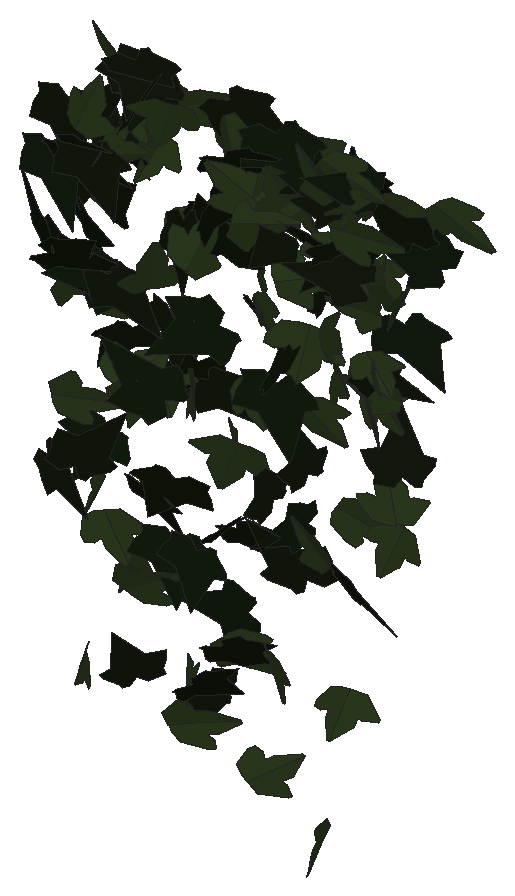
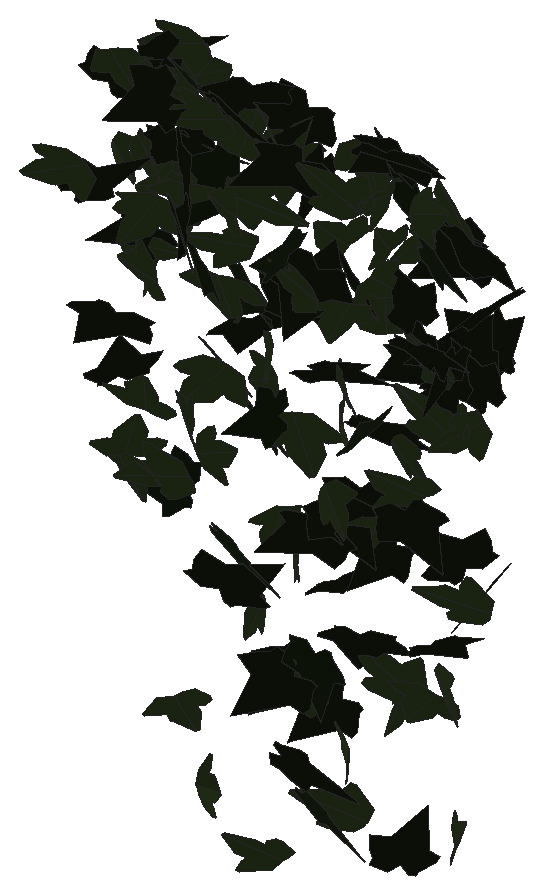
# SketchUp Ruby script. Lengths in inches.
U = 1.inch
M = Sketchup.active_model
def pt(a) = Geom::Point3d.new(a.map { |v| v * U })
def face(e, loops, mat)
  f = e.add_face(loops[0].map { |a| pt(a) })
  loops[1..].each { |l| e.add_face(l.map { |a| pt(a) }).erase! }
  f.material = f.back_material = mat if mat
  f
end
# faces: each face lists its corners as indices into pts; further lists are holes
def faces(e, pts, list, mat = nil) = list.each { |f| face(e, (f[0].is_a?(Array) ? f : [f]).map { |l| l.map { |i| pts[i] } }, mat) }
# xy, xz, yz: faces in a plane at the given z, y or x. An outline is a flat list of corners, or four numbers for a rectangle; further outlines are holes
def ring(l) = l.size == 4 ? [[l[0], l[1]], [l[2], l[1]], [l[2], l[3]], [l[0], l[3]]] : l.each_slice(2).to_a
def flat(e, list, mat, &to3) = list.each { |f| face(e, (f[0].is_a?(Array) ? f : [f]).map { |l| ring(l).map { |u, v| to3.(u, v) } }, mat) }
def xy(e, z, list, mat = nil) = flat(e, list, mat) { |x, y| [x, y, z] }
def xz(e, y, list, mat = nil) = flat(e, list, mat) { |x, z| [x, y, z] }
def yz(e, x, list, mat = nil) = flat(e, list, mat) { |y, z| [x, y, z] }
def lines(e, pts, list) = list.each { |a, b| e.add_line(pt(pts[a]), pt(pts[b])) }
# prism: a flat outline (further loops are holes) pulled along v
def prism(e, loops, v, mat = nil)
  f = face(e, loops, mat); d = Geom::Vector3d.new(v.map { |x| x * U })
  f.pushpull(f.normal.samedirection?(d) ? d.length : -d.length)
end
def box(e, o, s, mat = nil) = prism(e, [[o, [o[0] + s[0], o[1], o[2]], [o[0] + s[0], o[1] + s[1], o[2]], [o[0], o[1] + s[1], o[2]]]], [0, 0, s[2]], mat)
def at(x, y, z, deg = 0) = Geom::Transformation.translation(pt([x, y, z])) * Geom::Transformation.rotation(ORIGIN, Z_AXIS, deg.degrees)
def axes(o, x, y, z) = Geom::Transformation.new([*x, 0, *y, 0, *z, 0, *pt(o).to_a, 1])
def part(name) = M.definitions.add(name)
# library, detail: a bought-in or finely detailed component or shape, given as its bounding box
def library(name, o, s) = part(name).tap { |d| box(d.entities, o, s) }
def detail(e, o, s) = box(e.add_group.entities, o, s)
def put(e, d, t, mat = nil) = e.add_instance(d, t).tap { |i| i.material = mat if mat }
def group(e, t, mat = nil) = e.add_group.tap { |g| g.transformation = t; g.material = mat if mat }.entities
root = M.entities
M.materials.add("1026 AP 7946 SUNNY SIDE UP").color = [254, 231, 186]
M.materials.add("efeu1").color = [18, 25, 13]
M.materials.add("efeu2").color = [43, 57, 29]
c1 = part("ivyleaf_9")
p = [[1.54,2.16,1.25],[1.36,2.04,1.19],[-0.21,0.99,0.68],[-0.71,1.11,0.82],[-0.85,0.86,0.67],[-0.8,0.17,0.21],
  [-0.9,-0.01,0.1],[-0.67,-0.16,-0.02],[-0.08,-0.08,-0.05],[-0.03,-0.6,-0.4],[0.65,-0.88,-0.66],[0.83,-0.6,-0.49],
  [1.29,-0.42,-0.43],[1.8125,-0.07,-0.26],[1.21,0.44,0.15]]
faces(c1.entities,p,[[0,1,2,3,4,5,6,7,8,9,10,11,12,13,14]],"efeu1")
c2 = part("ivyleaf_10")
p = [[0,0.5,-0.03],[-0.0625,2.02,-0.43],[-0.19,2.01,-0.46],[-0.54,1.05,-0.29],[-0.52,0.625,-0.18],[-0.83,0.76,-0.28],
  [-1.16,0.64,-0.33],[-1.15,0.33,-0.24],[-0.77,-0.39,0.02],[-0.3,-0.51,0.16],[0.04,-0.48,0.23],[-0.02,2.01,-0.4375],
  [-0.06,2.01,-0.43],[0.04,-0.49,0.23],[0.67,-0.49,0.14],[1.38,0.36,-0.2],[1.375,0.51,-0.24],[0.81,0.65,-0.19],
  [0.62,0.59,-0.15],[0.6,1.09,-0.28],[0.5,1.23,-0.31]]
faces(c2.entities,p,[[0,1,2,3,4,5,6,7,8,9,10],[11,12,0,13,14,15,16,17,18,19,20]],"efeu2")
put(root,c1,axes([130.41,212.4,265.85],[-0.4161,-0.11399,-0.10586],[0.16625,0.01128,-0.29519],[0.17397,-0.28342,0.0289]),"1026 AP 7946 SUNNY SIDE UP")
put(root,c2,axes([130.06,211.54,261.31],[-0.09725,0.00024,0.32369],[0.41165,0.17712,0.05398],[-0.27319,0.26679,-0.03389]),"1026 AP 7946 SUNNY SIDE UP")
put(root,c1,axes([130.375,211.64,265.35],[0.10675,-0.1348,-0.29209],[-0.24694,0.23569,-0.15322],[0.42618,0.17033,-0.01562]),"1026 AP 7946 SUNNY SIDE UP")
put(root,c1,axes([130.58,210.33,264.84],[0.08748,-0.17485,0.29547],[-0.06631,0.28579,0.18894],[-0.52534,-0.06519,0.02535]),"1026 AP 7946 SUNNY SIDE UP")
put(root,c1,axes([130.27,210.95,265.93],[0.03924,-0.37961,-0.02403],[-0.00771,0.02089,-0.39177],[0.59777,0.02519,-0.00348]),"1026 AP 7946 SUNNY SIDE UP")
put(root,c1,axes([130.53,211.9,260.69],[-0.27687,-0.23897,0.07479],[-0.04522,-0.0705,-0.30564],[0.39072,-0.17749,0.01762]),"1026 AP 7946 SUNNY SIDE UP")
put(root,c2,axes([130.61,211.62,259.94],[0.18156,-0.29153,-0.01318],[-0.02473,0.00574,-0.32274],[0.45807,0.11586,-0.0122]),"1026 AP 7946 SUNNY SIDE UP")
put(root,c1,axes([130.5,211.02,266.875],[-0.3624,-0.07053,-0.28017],[0.42422,0.04074,-0.24655],[0.12108,-0.35384,0.02528]),"1026 AP 7946 SUNNY SIDE UP")
put(root,c2,axes([130.57,210.92,263.8125],[-0.10801,-0.11461,-0.30654],[0.27721,0.23918,-0.13574],[0.41664,-0.18885,0.01084]),"1026 AP 7946 SUNNY SIDE UP")
put(root,c1,axes([130.45,210.83,264.34],[-0.00135,-0.02148,0.32525],[0.23378,-0.27887,-0.02076],[0.43946,0.14828,0.01204]),"1026 AP 7946 SUNNY SIDE UP")
put(root,c2,axes([130.7,211.22,257.11],[-0.00482,0.04885,-0.30958],[0.02814,-0.30025,-0.05218],[-0.47832,-0.01815,0.00005]),"1026 AP 7946 SUNNY SIDE UP")
put(root,c2,axes([131.05,211.57,267.45],[-0.1691,0.14723,-0.26811],[-0.28544,0.18873,0.18778],[0.37504,0.21003,0.02203]),"1026 AP 7946 SUNNY SIDE UP")
put(root,c1,axes([130.53,211.39,264.57],[0.0731,-0.0828,0.29971],[0.1641,-0.27239,-0.09848],[0.44718,0.11349,-0.01286]),"1026 AP 7946 SUNNY SIDE UP")
put(root,c1,axes([130.66,210.38,260.98],[0.26146,-0.24764,-0.17909],[-0.15805,0.14018,-0.30643],[0.44739,0.19425,-0.00359]),"1026 AP 7946 SUNNY SIDE UP")
put(root,c1,axes([130.95,211.57,266.88],[-0.34929,0.13944,-0.16772],[0.18724,-0.11603,-0.26914],[-0.2814,-0.25029,0.02909]),"1026 AP 7946 SUNNY SIDE UP")
put(root,c2,axes([130.54,211.73,265.12],[0.15804,-0.09938,-0.30184],[0.37693,-0.16881,0.14299],[-0.30622,-0.25908,0.02023]),"1026 AP 7946 SUNNY SIDE UP")
put(root,c1,axes([131.03,211.89,262.68],[0.05808,0.21636,-0.21679],[-0.04333,-0.20995,-0.22726],[-0.47395,0.04571,-0.00579]),"1026 AP 7946 SUNNY SIDE UP")
put(root,c1,axes([130.96,211.5,265.05],[-0.0691,0.09761,0.31381],[0.12997,-0.29299,0.10749],[0.48503,0.09241,0.0159]),"1026 AP 7946 SUNNY SIDE UP")
put(root,c1,axes([130.88,210.49,266.46],[0.49526,0.04975,0.08038],[0.12809,-0.01989,-0.32702],[-0.06823,0.32381,-0.03049]),"1026 AP 7946 SUNNY SIDE UP")
put(root,c2,axes([130.93,211.46,259.47],[0.41877,0.11041,0.15008],[0.22928,0.02509,-0.29534],[-0.17203,0.30223,-0.02829]),"1026 AP 7946 SUNNY SIDE UP")
put(root,c1,axes([131.26,211.74,256.79],[0.21556,0.113,0.25928],[-0.36903,-0.09862,0.17719],[0.22627,-0.26849,0.04198]),"1026 AP 7946 SUNNY SIDE UP")
put(root,c2,axes([131.0625,210.69,266.91],[0.48737,-0.17816,-0.02697],[0.06055,0.01671,0.36677],[-0.27636,-0.31052,0.03279]),"1026 AP 7946 SUNNY SIDE UP")
put(root,c1,axes([130.88,210.16,264.72],[0.38747,0.12743,0.2176],[0.31784,0.06505,-0.28396],[-0.22064,0.31749,-0.02692]),"1026 AP 7946 SUNNY SIDE UP")
put(root,c1,axes([130.98,211.77,265.875],[-0.02801,-0.107,0.30558],[0.21146,-0.27195,-0.09414],[0.44947,0.12128,0.06333]),"1026 AP 7946 SUNNY SIDE UP")
put(root,c1,axes([131.41,210.9,264.16],[-0.01935,-0.24901,-0.22279],[0.01795,-0.21519,0.25501],[-0.51683,0.00185,0.0172]),"1026 AP 7946 SUNNY SIDE UP")
put(root,c2,axes([131.03,211.05,263.67],[-0.35983,-0.03803,0.26783],[0.39011,0.08311,0.23778],[-0.13705,0.3364,-0.02636]),"1026 AP 7946 SUNNY SIDE UP")
put(root,c1,axes([131.21,210.36,261.08],[-0.14586,-0.052,0.33939],[0.46342,0.14793,0.11032],[-0.24646,0.30894,0.00657]),"1026 AP 7946 SUNNY SIDE UP")
put(root,c1,axes([131.38,210.45,266.53],[-0.25841,-0.13518,-0.25909],[0.34512,0.1244,-0.21658],[0.28547,-0.27276,0.02731]),"1026 AP 7946 SUNNY SIDE UP")
put(root,c2,axes([131.66,211.14,259.14],[-0.0176,-0.21279,-0.25113],[0.08895,0.23765,-0.21607],[0.4995,-0.04982,0.02963]),"1026 AP 7946 SUNNY SIDE UP")
put(root,c2,axes([131.58,210.65,266.53],[-0.0774,-0.12712,-0.33864],[0.22425,0.29554,-0.13832],[0.50562,-0.15054,0.00951]),"1026 AP 7946 SUNNY SIDE UP")
put(root,c2,axes([131.75,211.73,266.22],[0.14936,0.20643,-0.24394],[-0.14698,-0.21889,-0.23533],[-0.47304,0.13319,-0.0039]),"1026 AP 7946 SUNNY SIDE UP")
put(root,c2,axes([131.74,211.4,266.59],[0.08454,0.22627,-0.21222],[0.07568,0.20162,0.24077],[0.47653,-0.07216,-0.00059]),"1026 AP 7946 SUNNY SIDE UP")
put(root,c2,axes([131.72,211.75,262.2],[0.25185,0.2614,0.02942],[0.04334,0.01482,-0.31532],[-0.41094,0.16176,-0.01523]),"1026 AP 7946 SUNNY SIDE UP")
put(root,c2,axes([131.58,211.03,262.4375],[0.33233,0.0674,-0.27773],[0.32476,0.18919,0.21633],[0.29321,-0.28594,0.07518]),"1026 AP 7946 SUNNY SIDE UP")
put(root,c1,axes([131.65,210.64,264.35],[-0.08789,-0.12663,-0.29627],[0.37113,0.17486,-0.12587],[0.32462,-0.23419,0.06369]),"1026 AP 7946 SUNNY SIDE UP")
put(root,c1,axes([131.8,210.81,267.12],[0.0186,0.30597,0.18253],[-0.03474,-0.17455,0.31412],[0.55349,-0.02124,0.01358]),"1026 AP 7946 SUNNY SIDE UP")
put(root,c1,axes([132.01,211.12,267.91],[-0.43255,-0.16604,-0.11611],[0.16644,0.04053,-0.3302],[0.26709,-0.29415,0.01774]),"1026 AP 7946 SUNNY SIDE UP")
put(root,c2,axes([132.09,212.33,262.77],[-0.00908,-0.30999,0.03736],[-0.00028,-0.03803,-0.31963],[0.49109,-0.00575,0.00051]),"1026 AP 7946 SUNNY SIDE UP")
put(root,c1,axes([132.18,212.06,262.42],[0.05336,0.20514,-0.23821],[-0.03048,-0.23192,-0.21517],[-0.48646,0.03703,-0.01265]),"1026 AP 7946 SUNNY SIDE UP")
put(root,c2,axes([132.31,210.39,262.6],[0.14838,-0.12751,-0.28872],[-0.30732,0.20072,-0.16112],[0.37276,0.21623,-0.01791]),"1026 AP 7946 SUNNY SIDE UP")
put(root,c1,axes([131.8125,211.07,267.97],[-0.10536,-0.14138,-0.28975],[0.34136,0.18638,-0.14914],[0.35689,-0.22001,0.05711]),"1026 AP 7946 SUNNY SIDE UP")
put(root,c2,axes([132.1,211.01,267.11],[0.11092,0.08744,-0.34608],[0.1092,0.33282,0.10607],[0.53556,-0.08597,0.05005]),"1026 AP 7946 SUNNY SIDE UP")
put(root,c2,axes([132.03,210.78,259.01],[-0.29475,-0.13307,0.22775],[0.30883,0.10507,0.23653],[-0.26472,0.27075,0.02236]),"1026 AP 7946 SUNNY SIDE UP")
put(root,c1,axes([132.15,211.53,263.38],[-0.00307,-0.2819,0.17273],[0.01518,-0.16925,-0.29126],[0.51682,0.0033,0.00958]),"1026 AP 7946 SUNNY SIDE UP")
put(root,c1,axes([132.82,210.42,262.76],[-0.47823,-0.14291,-0.09538],[-0.15201,-0.0091,0.34459],[-0.21957,0.31756,-0.03082]),"1026 AP 7946 SUNNY SIDE UP")
put(root,c1,axes([132.89,212.35,258.19],[-0.15848,-0.0612,-0.30212],[-0.43574,-0.09754,0.11866],[-0.17755,0.29401,-0.02154]),"1026 AP 7946 SUNNY SIDE UP")
put(root,c2,axes([132.69,210.77,267.56],[-0.42298,-0.17038,0.0685],[-0.06368,-0.06159,-0.32696],[0.28101,-0.27041,0.02902]),"1026 AP 7946 SUNNY SIDE UP")
put(root,c2,axes([132.6,210.47,264.7],[-0.25982,-0.32545,-0.05494],[-0.06113,-0.03794,0.37537],[-0.51448,0.16887,-0.01685]),"1026 AP 7946 SUNNY SIDE UP")
put(root,c1,axes([132.72,211.9,259.73],[0.02197,0.3089,0.04449],[0.0038,0.04136,-0.31831],[-0.49005,0.01417,-0.00047]),"1026 AP 7946 SUNNY SIDE UP")
put(root,c1,axes([132.51,211.13,259.81],[-0.30636,-0.22212,-0.14381],[0.16937,0.08911,-0.30315],[0.37498,-0.22172,0.01943]),"1026 AP 7946 SUNNY SIDE UP")
put(root,c1,axes([132.42,210.47,261.03],[0.48773,-0.04911,-0.06379],[-0.10306,-0.02178,-0.32206],[0.06881,0.3155,-0.03026]),"1026 AP 7946 SUNNY SIDE UP")
put(root,c2,axes([132.27,212.68,266.21],[0.03557,-0.04582,-0.32016],[0.38276,-0.19398,0.04662],[-0.31158,-0.24353,0.02072]),"1026 AP 7946 SUNNY SIDE UP")
put(root,c1,axes([132.33,212.22,262.07],[-0.03293,-0.04917,-0.31645],[0.27613,0.25192,-0.05246],[0.40325,-0.17652,0.01007]),"1026 AP 7946 SUNNY SIDE UP")
put(root,c2,axes([132.37,211.58,267.18],[-0.2953,-0.10107,0.2563],[0.34442,0.11919,0.22041],[-0.24572,0.28853,0.00092]),"1026 AP 7946 SUNNY SIDE UP")
put(root,c2,axes([132.51,211.46,265.32],[0.31369,0.25213,0.06884],[0.08881,0.03853,-0.33035],[-0.39982,0.20637,-0.01937]),"1026 AP 7946 SUNNY SIDE UP")
put(root,c1,axes([133.03,211.66,257.16],[-0.36348,0.21185,-0.00052],[-0.02394,-0.01914,-0.32216],[-0.33227,-0.23038,0.02379]),"1026 AP 7946 SUNNY SIDE UP")
put(root,c2,axes([133.02,210.82,257.56],[0.1482,-0.07138,0.30828],[-0.30747,0.22826,0.12071],[-0.37424,-0.2158,0.0229]),"1026 AP 7946 SUNNY SIDE UP")
put(root,c2,axes([132.75,211.23,263.91],[0.25979,-0.20189,0.17712],[0.1677,-0.13635,-0.26953],[0.38304,0.19662,-0.00213]),"1026 AP 7946 SUNNY SIDE UP")
put(root,c1,axes([132.6875,212.59,266.65],[0.23118,-0.28935,0.04424],[0.0138,-0.04552,-0.33437],[0.46014,0.14674,-0.0122]),"1026 AP 7946 SUNNY SIDE UP")
put(root,c2,axes([133.08,211.86,261.35],[0.06204,-0.05587,-0.31638],[-0.10254,0.30092,-0.06334],[0.47949,0.07158,0.02739]),"1026 AP 7946 SUNNY SIDE UP")
put(root,c1,axes([132.83,210.92,265.59],[-0.27125,-0.04021,-0.334],[0.50387,-0.09093,-0.16468],[-0.09817,-0.35561,0.07763]),"1026 AP 7946 SUNNY SIDE UP")
put(root,c1,axes([132.79,212.375,259.58],[0.46167,0.1039,0.04642],[0.07971,-0.01044,-0.31975],[-0.15882,0.29677,-0.02554]),"1026 AP 7946 SUNNY SIDE UP")
put(root,c2,axes([132.74,211.04,256.74],[-0.16689,-0.05706,0.31377],[0.34928,0.21095,0.12156],[-0.34045,0.24439,-0.0291]),"1026 AP 7946 SUNNY SIDE UP")
put(root,c1,axes([133.2,210.23,261.54],[0.26151,0.14073,-0.24852],[-0.24939,-0.18463,-0.22395],[-0.36278,0.22836,-0.0252]),"1026 AP 7946 SUNNY SIDE UP")
put(root,c1,axes([133.32,211.1,263.88],[-0.42724,-0.14345,0.16641],[-0.18813,-0.11773,-0.31415],[0.28398,-0.29381,0.04224]),"1026 AP 7946 SUNNY SIDE UP")
put(root,c2,axes([132.99,212.28,262.16],[0.11557,0.29731,0.07959],[0.04846,0.07016,-0.31482],[-0.47991,0.07868,-0.01262]),"1026 AP 7946 SUNNY SIDE UP")
put(root,c1,axes([133.05,211.47,265.75],[0.38204,0.2658,-0.01925],[0.00399,-0.02962,-0.37048],[-0.41914,0.24199,-0.02107]),"1026 AP 7946 SUNNY SIDE UP")
put(root,c1,axes([133.21,211.39,265.02],[0.48064,-0.02938,0.24623],[-0.36139,0.08059,0.31327],[-0.1139,-0.37967,0.04511]),"1026 AP 7946 SUNNY SIDE UP")
put(root,c2,axes([133.51,211.98,264.51],[-0.01454,0.03064,0.32089],[-0.29981,0.24635,-0.02938],[-0.38994,-0.19055,0.01062]),"1026 AP 7946 SUNNY SIDE UP")
put(root,c2,axes([133.12,210.76,262.89],[0.0281,-0.02911,0.33384],[0.34019,-0.24156,-0.03604],[0.38245,0.21701,0.00753]),"1026 AP 7946 SUNNY SIDE UP")
put(root,c1,axes([133.375,210.57,260.18],[-0.13633,-0.29958,0.03071],[0.00546,-0.03378,-0.32122],[0.47362,-0.08584,0.01254]),"1026 AP 7946 SUNNY SIDE UP")
put(root,c1,axes([133.17,212.22,263.67],[0.4052,-0.17636,0.03924],[0.02801,-0.04296,-0.32089],[0.28265,0.25708,-0.02445]),"1026 AP 7946 SUNNY SIDE UP")
put(root,c1,axes([133.25,211.59,267.55],[-0.01019,-0.0632,-0.3339],[0.22433,0.29143,-0.05985],[0.46766,-0.14117,0.02143]),"1026 AP 7946 SUNNY SIDE UP")
put(root,c2,axes([133.52,210.22,265.53],[0.17944,0.2392,-0.30207],[0.16449,0.27585,0.27412],[0.57354,-0.15395,0.01589]),"1026 AP 7946 SUNNY SIDE UP")
put(root,c1,axes([133.53,210.33,258.04],[0.26314,0.23417,0.15756],[0.17496,0.1061,-0.29472],[-0.40225,0.19934,-0.02511]),"1026 AP 7946 SUNNY SIDE UP")
put(root,c2,axes([133.7,210.96,267.52],[-0.05578,0.3459,-0.05384],[0.00149,-0.05441,-0.3585],[-0.55054,-0.03519,0.00448]),"1026 AP 7946 SUNNY SIDE UP")
put(root,c2,axes([133.6,211.87,264.01],[-0.22527,0.13914,-0.24809],[0.21191,-0.20323,-0.20409],[-0.38378,-0.19389,0.03293]),"1026 AP 7946 SUNNY SIDE UP")
put(root,c1,axes([133.99,210.15,266.64],[0.0285,-0.01812,-0.38175],[-0.37753,0.28213,-0.02467],[0.44453,0.24077,0.00352]),"1026 AP 7946 SUNNY SIDE UP")
put(root,c1,axes([133.8,210.74,258.6],[0.39758,0.18668,0.08523],[0.12797,0.02681,-0.32253],[-0.29373,0.26436,-0.02514]),"1026 AP 7946 SUNNY SIDE UP")
put(root,c2,axes([133.74,211.62,255.95],[0.2673,0.05464,-0.26674],[0.34073,0.14853,0.17951],[0.23966,-0.2721,0.04229]),"1026 AP 7946 SUNNY SIDE UP")
put(root,c2,axes([133.77,211.01,258.53],[-0.29965,-0.08892,-0.26334],[0.38722,0.07124,-0.21467],[0.17474,-0.31037,0.02411]),"1026 AP 7946 SUNNY SIDE UP")
put(root,c2,axes([134.41,211.39,266.45],[0.12216,-0.00267,-0.33541],[-0.51194,-0.00016,-0.08004],[0.00072,0.33471,-0.00075]),"1026 AP 7946 SUNNY SIDE UP")
put(root,c2,axes([134.27,210.41,262.33],[-0.49407,-0.14099,0.10777],[-0.12089,-0.08411,-0.35247],[0.24901,-0.32057,0.04271]),"1026 AP 7946 SUNNY SIDE UP")
put(root,c1,axes([134.21,210.25,267.5],[0.3711,0.24176,0.02984],[0.05655,0.00337,-0.34721],[-0.37841,0.23759,-0.02262]),"1026 AP 7946 SUNNY SIDE UP")
put(root,c2,axes([134.46,210.64,266.94],[0.31201,-0.17988,0.29658],[-0.29669,0.22018,0.27602],[-0.44537,-0.27269,0.0239]),"1026 AP 7946 SUNNY SIDE UP")
put(root,c2,axes([134.46,210.45,266.85],[0.14517,0.28951,0.22768],[-0.12062,-0.20569,0.31173],[0.55826,-0.11973,0.00815]),"1026 AP 7946 SUNNY SIDE UP")
put(root,c1,axes([134.79,211.45,260.78],[-0.4013,0.18684,-0.029],[0.01022,-0.04036,-0.32475],[-0.29718,-0.25369,0.02799]),"1026 AP 7946 SUNNY SIDE UP")
put(root,c1,axes([134.83,211.39,259.9],[0.11468,0.02942,0.32943],[-0.48231,0.10287,0.06296],[-0.14856,-0.31126,0.04991]),"1026 AP 7946 SUNNY SIDE UP")
put(root,c1,axes([134.95,212.37,266.51],[-0.07547,-0.01441,-0.32793],[-0.46104,0.12784,0.04034],[0.19586,0.29536,-0.03141]),"1026 AP 7946 SUNNY SIDE UP")
put(root,c2,axes([134.49,210.33,266.46],[-0.05497,-0.0693,-0.37138],[0.36822,0.27415,-0.07617],[0.44373,-0.23608,0.0172]),"1026 AP 7946 SUNNY SIDE UP")
put(root,c2,axes([134.47,211.6,266.28],[0.06108,-0.04059,0.33834],[0.45667,-0.15481,-0.05596],[0.25018,0.2925,0.01956]),"1026 AP 7946 SUNNY SIDE UP")
put(root,c1,axes([134.59,212.54,266.43],[0.07142,-0.05116,-0.32444],[0.45239,-0.13028,0.06385],[-0.21584,-0.28999,0.02646]),"1026 AP 7946 SUNNY SIDE UP")
put(root,c1,axes([134.85,210.82,266.16],[-0.13273,-0.21486,0.25811],[-0.13037,-0.23781,-0.23911],[0.50385,-0.11814,0.00613]),"1026 AP 7946 SUNNY SIDE UP")
put(root,c2,axes([134.99,210.76,266.9],[-0.21949,-0.25782,-0.19431],[-0.16476,-0.15581,0.30072],[-0.47307,0.17388,-0.01457]),"1026 AP 7946 SUNNY SIDE UP")
put(root,c1,axes([135.3,210.79,267.35],[-0.19619,0.19961,0.25733],[-0.28698,0.17424,-0.23742],[-0.41113,-0.21688,0.04293]),"1026 AP 7946 SUNNY SIDE UP")
put(root,c2,axes([134.68,212.3,262.97],[-0.05178,0.06873,0.3513],[0.42645,-0.2088,0.06919],[0.34156,0.27111,-0.03314]),"1026 AP 7946 SUNNY SIDE UP")
put(root,c1,axes([135.27,210.04,262.02],[-0.30301,0.06467,-0.26935],[-0.35951,0.13149,0.20759],[0.22491,0.29731,-0.03106]),"1026 AP 7946 SUNNY SIDE UP")
put(root,c1,axes([134.8125,210.76,267.87],[-0.104,-0.26807,-0.25118],[0.13758,0.22711,-0.28213],[0.55127,-0.10725,0.02303]),"1026 AP 7946 SUNNY SIDE UP")
put(root,c2,axes([135.1,210.26,259.05],[-0.3353,0.23436,-0.03572],[0.01173,-0.04176,-0.32584],[-0.37265,-0.21219,0.02188]),"1026 AP 7946 SUNNY SIDE UP")
put(root,c1,axes([135.32,210.16,264.1875],[-0.26808,0.13146,-0.24321],[-0.26769,0.16566,0.22195],[0.33128,0.24024,-0.01747]),"1026 AP 7946 SUNNY SIDE UP")
put(root,c1,axes([135.375,211.25,265.07],[-0.00979,0.19059,0.36138],[-0.05685,0.34804,-0.19404],[-0.62366,-0.03471,0.01202]),"1026 AP 7946 SUNNY SIDE UP")
put(root,c2,axes([134.87,210.9375,265.32],[0.1626,-0.02698,-0.32558],[0.43347,0.17175,0.07886],[0.2462,-0.28457,0.07618]),"1026 AP 7946 SUNNY SIDE UP")
put(root,c1,axes([135.09,210.38,263.77],[-0.13118,-0.3416,-0.10883],[0.04518,0.09972,-0.36165],[0.55952,-0.08814,0.00369]),"1026 AP 7946 SUNNY SIDE UP")
put(root,c1,axes([135.09,210.76,266.35],[0.54164,0.04815,-0.08028],[-0.13379,0.0531,-0.35212],[-0.05434,0.34922,0.06674]),"1026 AP 7946 SUNNY SIDE UP")
put(root,c2,axes([135.29,210.82,264.51],[0.56752,0.04571,-0.01108],[-0.01028,-0.03562,-0.37331],[-0.07321,0.35933,-0.03344]),"1026 AP 7946 SUNNY SIDE UP")
put(root,c2,axes([135.21,211.03,263.14],[-0.41988,-0.09212,-0.1833],[0.27629,0.03298,-0.28992],[0.14987,-0.31889,0.02093]),"1026 AP 7946 SUNNY SIDE UP")
put(root,c1,axes([135.62,211.31,266.38],[0.05328,-0.09922,0.39594],[0.00631,0.38636,0.1045],[-0.62496,-0.00456,0.03481]),"1026 AP 7946 SUNNY SIDE UP")
put(root,c2,axes([135.48,211.59,257.9],[0.31622,0.21738,-0.12582],[-0.11329,-0.10121,-0.3053],[-0.37633,0.21312,-0.01382]),"1026 AP 7946 SUNNY SIDE UP")
put(root,c2,axes([135.12,211.24,267.46],[0.20468,0.07704,0.30651],[0.44003,0.10271,-0.15315],[-0.19815,0.30766,-0.0235]),"1026 AP 7946 SUNNY SIDE UP")
put(root,c2,axes([135.5625,212.26,263.04],[0.50497,0.03427,0.02951],[-0.05276,0.04988,0.32851],[0.04607,-0.31852,0.05268]),"1026 AP 7946 SUNNY SIDE UP")
put(root,c2,axes([135.6,211.17,266.07],[0.46375,0.13064,-0.01119],[-0.00051,-0.02783,-0.33145],[-0.20622,0.29385,-0.02434]),"1026 AP 7946 SUNNY SIDE UP")
put(root,c1,axes([135.93,210.08,262.7],[-0.35484,0.1029,-0.17199],[-0.22908,0.08375,0.25564],[0.20761,0.26829,-0.01188]),"1026 AP 7946 SUNNY SIDE UP")
put(root,c2,axes([135.99,210.375,267.52],[-0.26158,0.11082,-0.26257],[-0.28958,0.17948,0.20478],[0.32849,0.24646,-0.02856]),"1026 AP 7946 SUNNY SIDE UP")
put(root,c2,axes([136.05,210.22,261.18],[-0.21182,0.10298,-0.25955],[-0.3009,0.16498,0.17544],[0.30553,0.23388,-0.00716]),"1026 AP 7946 SUNNY SIDE UP")
put(root,c2,axes([135.71,210.71,256.01],[0.13576,-0.16043,0.29014],[0.19114,-0.25517,-0.18902],[0.47379,0.14891,-0.00688]),"1026 AP 7946 SUNNY SIDE UP")
put(root,c1,axes([136.3,210.36,267.38],[-0.27707,0.22979,0.10818],[-0.133,0.06531,-0.29675],[-0.37344,-0.19375,0.02542]),"1026 AP 7946 SUNNY SIDE UP")
put(root,c1,axes([136.33,210.51,266.49],[0.05462,0.15795,-0.28197],[-0.06085,-0.27206,-0.16785],[-0.49438,0.05093,-0.01049]),"1026 AP 7946 SUNNY SIDE UP")
put(root,c2,axes([135.8,211.28,261.36],[0.17836,0.04706,0.32675],[0.44581,0.14182,-0.12541],[-0.23461,0.30526,0.0101]),"1026 AP 7946 SUNNY SIDE UP")
put(root,c2,axes([136.25,210.14,265.18],[-0.08926,0.21549,0.21482],[-0.12119,0.19333,-0.22764],[-0.45428,-0.09391,0.01852]),"1026 AP 7946 SUNNY SIDE UP")
put(root,c2,axes([136.14,211.37,265.7],[-0.31788,-0.2074,-0.18066],[0.24563,0.08828,-0.29454],[0.3479,-0.25183,0.04289]),"1026 AP 7946 SUNNY SIDE UP")
put(root,c1,axes([135.98,211.22,267.53],[0.49426,-0.06911,0.0461],[0.05773,-0.04215,-0.33006],[0.11625,0.31475,-0.03212]),"1026 AP 7946 SUNNY SIDE UP")
put(root,c1,axes([136.69,210.33,266.15],[-0.28283,0.07489,0.23098],[-0.35927,0.01509,-0.19431],[-0.09278,-0.28671,0.04831]),"1026 AP 7946 SUNNY SIDE UP")
put(root,c1,axes([136.11,212.26,264.34],[-0.15861,-0.18091,-0.25977],[0.26159,0.19104,-0.2095],[0.41039,-0.19169,0.03314]),"1026 AP 7946 SUNNY SIDE UP")
put(root,c1,axes([136.7,210.57,267.64],[-0.12904,-0.02204,0.29895],[-0.39453,-0.14764,-0.08548],[0.23221,-0.26309,0.02089]),"1026 AP 7946 SUNNY SIDE UP")
put(root,c2,axes([136.5,210.77,265.67],[0.06741,0.15538,-0.34053],[0.0573,0.33023,0.16628],[0.57272,-0.05133,0.02345]),"1026 AP 7946 SUNNY SIDE UP")
put(root,c2,axes([136.19,210.43,267.96],[-0.23154,-0.02082,-0.28816],[0.43475,-0.06316,-0.14554],[-0.07311,-0.30962,0.04717]),"1026 AP 7946 SUNNY SIDE UP")
put(root,c2,axes([136.53,211.42,261.62],[0.34407,0.25251,-0.00616],[-0.01762,0.0195,0.34364],[0.39683,-0.21807,0.0206]),"1026 AP 7946 SUNNY SIDE UP")
put(root,c1,axes([136.18,210.57,260.72],[0.33862,-0.19813,0.16439],[0.15882,-0.12689,-0.30137],[0.36835,0.23685,-0.02118]),"1026 AP 7946 SUNNY SIDE UP")
put(root,c2,axes([136.91,210.33,265.73],[0.0576,0.0047,-0.26956],[-0.39734,0.06947,-0.03475],[0.1072,0.25495,0.01604]),"1026 AP 7946 SUNNY SIDE UP")
put(root,c2,axes([136.75,210.62,267.49],[-0.02143,-0.15711,0.25673],[-0.01624,-0.24996,-0.1638],[0.46413,-0.016,0.00612]),"1026 AP 7946 SUNNY SIDE UP")
put(root,c2,axes([136.97,210.6,266.09],[-0.18794,0.10027,0.25884],[-0.36839,0.09774,-0.15478],[-0.21101,-0.25996,0.03968]),"1026 AP 7946 SUNNY SIDE UP")
put(root,c2,axes([136.7,211.29,261.32],[0.50441,-0.12086,-0.01201],[-0.03351,-0.02558,-0.35182],[0.18786,0.31996,-0.03051]),"1026 AP 7946 SUNNY SIDE UP")
put(root,c1,axes([137.07,211.84,265.89],[-0.05978,0.02577,0.33129],[-0.45291,-0.14823,-0.02372],[0.22796,-0.28774,0.03975]),"1026 AP 7946 SUNNY SIDE UP")
put(root,c1,axes([136.9375,211.13,262.57],[-0.32225,-0.15786,0.22872],[0.27181,0.14081,0.26728],[-0.33254,0.26807,-0.00317]),"1026 AP 7946 SUNNY SIDE UP")
put(root,c2,axes([137.24,210.41,264.33],[-0.04097,0.00703,-0.28497],[-0.42912,0.04547,0.02794],[0.07222,0.27413,0.00433]),"1026 AP 7946 SUNNY SIDE UP")
put(root,c2,axes([136.5,210.25,267.01],[-0.11932,-0.00781,0.37378],[0.56017,0.0693,0.07869],[-0.10916,0.36418,-0.00475]),"1026 AP 7946 SUNNY SIDE UP")
put(root,c2,axes([136.93,210.35,264.04],[-0.19496,0.25593,-0.02975],[0.00208,-0.03303,-0.29285],[-0.40523,-0.1233,0.01281]),"1026 AP 7946 SUNNY SIDE UP")
put(root,c2,axes([136.7,210.68,264.06],[0.11661,-0.00587,0.36144],[0.51528,-0.12716,-0.07429],[0.19744,0.33534,-0.01959]),"1026 AP 7946 SUNNY SIDE UP")
put(root,c2,axes([137.12,210.28,264.79],[-0.10161,0.22412,0.11015],[-0.07832,0.0952,-0.23888],[-0.38164,-0.07921,0.0197]),"1026 AP 7946 SUNNY SIDE UP")
put(root,c2,axes([136.84,212.34,266.55],[-0.30955,-0.0222,-0.27063],[0.41184,-0.05238,-0.19805],[-0.04538,-0.32396,0.04861]),"1026 AP 7946 SUNNY SIDE UP")
put(root,c2,axes([137.25,210.78,267.5],[0.38394,0.05873,-0.1336],[-0.22177,0.06057,-0.24433],[-0.03378,0.26992,0.08564]),"1026 AP 7946 SUNNY SIDE UP")
put(root,c1,axes([136.94,210.37,264.63],[0.03486,0.01979,-0.26697],[0.1829,0.23195,0.02985],[0.36565,-0.11791,0.01052]),"1026 AP 7946 SUNNY SIDE UP")
put(root,c1,axes([137.45,210.68,267.02],[0.11549,-0.01316,0.28036],[-0.38462,0.12114,0.07474],[-0.18897,-0.2546,0.01923]),"1026 AP 7946 SUNNY SIDE UP")
put(root,c2,axes([137.03,210.25,264.94],[0.31275,0.11711,0.12047],[0.16899,0.04626,-0.23713],[-0.19691,0.2257,-0.01218]),"1026 AP 7946 SUNNY SIDE UP")
put(root,c2,axes([137.28,210.7,265.96],[0.10214,-0.25915,0.07616],[0.02194,-0.07422,-0.27563],[0.42382,0.0663,-0.00408]),"1026 AP 7946 SUNNY SIDE UP")
